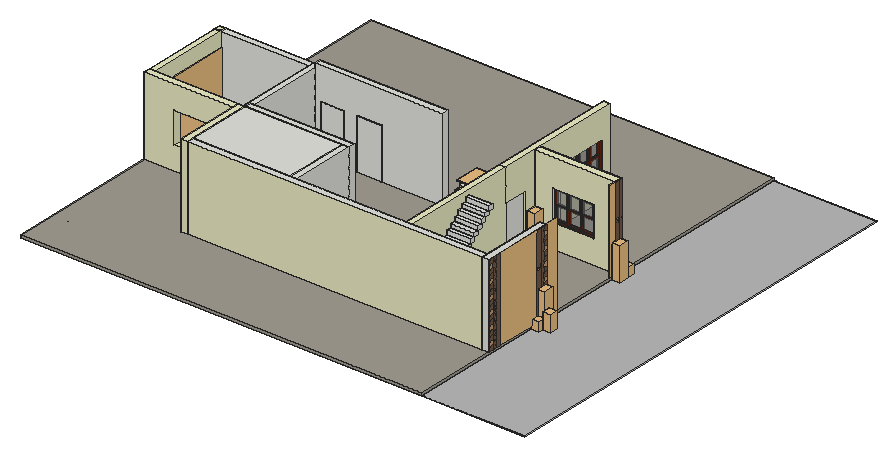
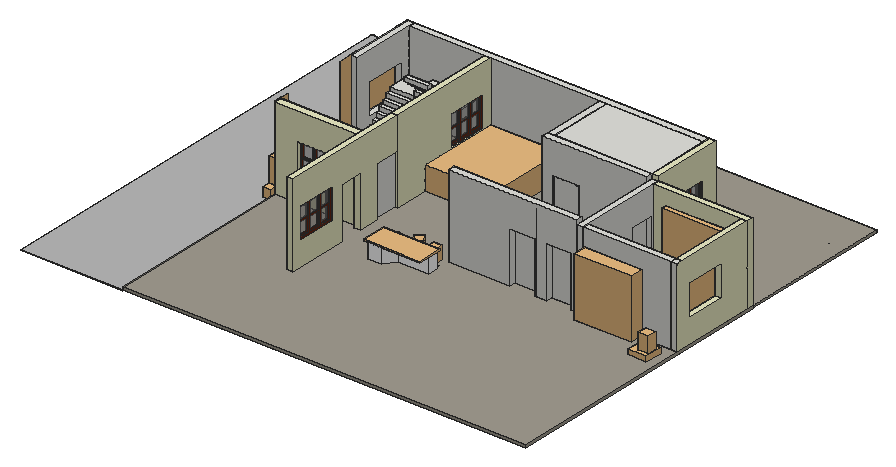
# SketchUp Ruby script. Lengths in inches.
U = 1.inch
M = Sketchup.active_model
def pt(a) = Geom::Point3d.new(a.map { |v| v * U })
def face(e, loops, mat)
  f = e.add_face(loops[0].map { |a| pt(a) })
  loops[1..].each { |l| e.add_face(l.map { |a| pt(a) }).erase! }
  f.material = f.back_material = mat if mat
  f
end
# faces: each face lists its corners as indices into pts; further lists are holes
def faces(e, pts, list, mat = nil) = list.each { |f| face(e, (f[0].is_a?(Array) ? f : [f]).map { |l| l.map { |i| pts[i] } }, mat) }
# xy, xz, yz: faces in a plane at the given z, y or x. An outline is a flat list of corners, or four numbers for a rectangle; further outlines are holes
def ring(l) = l.size == 4 ? [[l[0], l[1]], [l[2], l[1]], [l[2], l[3]], [l[0], l[3]]] : l.each_slice(2).to_a
def flat(e, list, mat, &to3) = list.each { |f| face(e, (f[0].is_a?(Array) ? f : [f]).map { |l| ring(l).map { |u, v| to3.(u, v) } }, mat) }
def xy(e, z, list, mat = nil) = flat(e, list, mat) { |x, y| [x, y, z] }
def xz(e, y, list, mat = nil) = flat(e, list, mat) { |x, z| [x, y, z] }
def yz(e, x, list, mat = nil) = flat(e, list, mat) { |y, z| [x, y, z] }
def lines(e, pts, list) = list.each { |a, b| e.add_line(pt(pts[a]), pt(pts[b])) }
# prism: a flat outline (further loops are holes) pulled along v
def prism(e, loops, v, mat = nil)
  f = face(e, loops, mat); d = Geom::Vector3d.new(v.map { |x| x * U })
  f.pushpull(f.normal.samedirection?(d) ? d.length : -d.length)
end
def box(e, o, s, mat = nil) = prism(e, [[o, [o[0] + s[0], o[1], o[2]], [o[0] + s[0], o[1] + s[1], o[2]], [o[0], o[1] + s[1], o[2]]]], [0, 0, s[2]], mat)
def at(x, y, z, deg = 0) = Geom::Transformation.translation(pt([x, y, z])) * Geom::Transformation.rotation(ORIGIN, Z_AXIS, deg.degrees)
def axes(o, x, y, z) = Geom::Transformation.new([*x, 0, *y, 0, *z, 0, *pt(o).to_a, 1])
def part(name) = M.definitions.add(name)
# library, detail: a bought-in or finely detailed component or shape, given as its bounding box
def library(name, o, s) = part(name).tap { |d| box(d.entities, o, s) }
def detail(e, o, s) = box(e.add_group.entities, o, s)
def put(e, d, t, mat = nil) = e.add_instance(d, t).tap { |i| i.material = mat if mat }
def group(e, t, mat = nil) = e.add_group.tap { |g| g.transformation = t; g.material = mat if mat }.entities
root = M.entities
M.materials.add("02 - Default1").color = [198, 154, 113]
M.materials.add("1").color = [234, 234, 196]
M.materials.add("3").color = [118, 89, 74]
M.materials.add("6").color = [162, 157, 145]
M.materials.add("Material1 glass").color = [170, 237, 177]
M.materials["Material1 glass"].alpha = 0.04
M.materials.add("Material1 metal").color = [192, 192, 192]
M.materials.add("[0080_DarkCyan]").color = [185, 185, 185]
M.materials.add("[Carpet_Plush_Charcoal]1").color = [87, 87, 87]
M.materials.add("[Color_004]1").color = [142, 142, 142]
M.materials.add("[Color_005]").color = [114, 114, 114]
M.materials.add("[Color_B17]").color = [102, 40, 20]
M.materials.add("[Tile_Ceramic_Natural]").color = [73, 73, 73]
M.materials.add("[Tile_Ceramic_Natural]1").color = [234, 234, 234]
M.materials.add("[Translucent_Glass_Gray]").color = [128, 128, 128]
M.materials["[Translucent_Glass_Gray]"].alpha = 0.5
M.materials.add("[Wood_ Floor]").color = [155, 105, 61]
M.materials.add("[Wood_Lumber_ButtJoined]").color = [69, 62, 43]
M.materials.add("putih ceramic").color = [255, 255, 255]
c1 = part("Group\#331")
xy(c1.entities,0,[[0,0,0.82,6.2]],"1")
xy(c1.entities,114.11,[[0,0,0.82,6.2]],"1")
xz(c1.entities,0,[[0,0,0.82,114.11]],"1")
xz(c1.entities,6.2,[[0,0,0.82,114.11]],"1")
yz(c1.entities,0,[[0,0,6.2,114.11]],"1")
yz(c1.entities,0.82,[[0,0,6.2,114.11]],"3")
c2 = part("Group\#330")
put(c2.entities,c1,axes([-0.82,0,0],[1,0,0],[0,1.45243,0],[0,0,1]),"1")
c3 = part("Group\#329")
box(c3.entities,[0,0,0],[0.82,6.2,114.11],"02 - Default1")
c4 = part("Group\#328")
put(c4.entities,c3,axes([-0.82,0,0],[1,0,0],[0,1.45243,0],[0,0,1]))
c5 = part("Group\#286")
put(c5.entities,c2,axes([0.82,0,0],[1,0,0],[0,0.6885,0],[0,0,1]),"02 - Default1")
put(c5.entities,c2,axes([0.82,6.2,89.22],[1,0,0],[0,0,0.67033],[0,-0.05434,0]),"02 - Default1")
put(c5.entities,c2,axes([0.82,6.2,12.68],[1,0,0],[0,0,0.67033],[0,-0.05434,0]),"02 - Default1")
put(c5.entities,c4,axes([0.82,6.2,63.7],[1,0,0],[0,0,0.67033],[0,-0.05434,0]),"02 - Default1")
put(c5.entities,c4,axes([0.82,6.2,25.75],[1,0,0],[0,0,0.67033],[0,-0.05434,0]),"02 - Default1")
put(c5.entities,c4,axes([0.82,6.2,82.99],[1,0,0],[0,0,0.67033],[0,-0.05434,0]),"02 - Default1")
put(c5.entities,c2,axes([0.82,6.2,50.83],[1,0,0],[0,0,0.67033],[0,-0.05434,0]),"02 - Default1")
put(c5.entities,c2,axes([0.82,6.2,76.54],[1,0,0],[0,0,0.67033],[0,-0.05434,0]),"02 - Default1")
put(c5.entities,c2,axes([0.82,6.2,31.98],[1,0,0],[0,0,0.67033],[0,-0.05434,0]),"02 - Default1")
put(c5.entities,c4,axes([0.82,6.2,44.6],[1,0,0],[0,0,0.67033],[0,-0.05434,0]),"02 - Default1")
g1 = group(c5.entities,at(0.82,6.2,95.39),"02 - Default1")
put(g1,c1,axes([-0.82,0,0],[1,0,0],[0,0,0.97361],[0,-0.05434,0]),"1")
put(c5.entities,c4,axes([0.82,6.2,101.84],[1,0,0],[0,0,0.67033],[0,-0.05434,0]),"02 - Default1")
put(c5.entities,c2,axes([0.82,6.2,0],[1,0,0],[0,0,0.67033],[0,-0.05434,0]),"02 - Default1")
put(c5.entities,c2,axes([0.82,6.2,19.3],[1,0,0],[0,0,0.67033],[0,-0.05434,0]),"02 - Default1")
put(c5.entities,c2,axes([0.82,6.2,69.93],[1,0,0],[0,0,0.67033],[0,-0.05434,0]),"02 - Default1")
put(c5.entities,c4,axes([0.82,6.2,6.45],[1,0,0],[0,0,0.67033],[0,-0.05434,0]),"02 - Default1")
put(c5.entities,c2,axes([0.82,6.2,38.15],[1,0,0],[0,0,0.67033],[0,-0.05434,0]),"02 - Default1")
put(c5.entities,c2,axes([0.82,6.2,57.25],[1,0,0],[0,0,0.67033],[0,-0.05434,0]),"02 - Default1")
put(c5.entities,c2,axes([0.82,6.2,108.07],[1,0,0],[0,0,0.67033],[0,-0.05434,0]),"02 - Default1")
c6 = library("Group\#185",[0,0,0],[15.75,57.83,12.57])
c7 = library("Group\#183",[0,0,0],[15.75,57.83,12.57])
c8 = library("Toilet",[49.48,5.86,0],[19.92,29.67,40.01])
c9 = library("Group\#134",[0,0,0],[3.17,3.17,3.01])
c10 = part("Framed panel")
g2 = group(c10.entities,at(0,0,0))
prism(g2,[[[0,22.64,0],[21.26,22.64,0],[21.26,0,0],[0,0,0]],[[1.57,1.57,0],[19.69,1.57,0],[19.69,21.0625,0],[1.57,21.0625,0]]],[0,0,1.57],"[Color_B17]")
g3 = group(c10.entities,at(1.57,1.57,1.02))
xy(g3,0,[[0,0,18.11,19.49]],"[Translucent_Glass_Gray]")
c11 = part("Group\#25")
put(c11.entities,c10,at(0,21.0625,1.57))
put(c11.entities,c10,at(0,0,0))
c12 = part("Group\#47")
g4 = group(c12.entities,at(0,0,0))
prism(g4,[[[70.87,0,0],[0,0,0],[0,47.24,0],[70.87,47.24,0]],[[47.83,1.77,0],[69.09,1.77,0],[69.09,45.47,0],[47.83,45.47,0]],[[46.0625,45.47,0],[24.8,45.47,0],[24.8,1.77,0],[46.0625,1.77,0]],[[1.77,1.77,0],[23.03,1.77,0],[23.03,45.47,0],[1.77,45.47,0]]],[0,0,4.33],"[Color_B17]")
put(c12.entities,c11,at(1.77,1.77,0.59))
put(c12.entities,c11,at(24.8,1.77,0.59))
put(c12.entities,c11,at(47.83,1.77,0.59))
c13 = library("Group\#332",[0,0,0],[0.82,72.71,126.79])
c14 = part("Group\#195")
box(c14.entities,[0,-29,0],[36,36,6])
c15 = part("Group\#196")
box(c15.entities,[0,0,0],[36,7,6])
c16 = part("Group\#197")
box(c16.entities,[0,0,0],[36,7,6])
c17 = part("Group\#165")
xy(c17.entities,0,[[3.14,0.77,2.7,0.83,2.28,1,1.93,1.27,1.65,1.63,1.48,2.04,4.8,2.93,4.86,2.49,4.8,2.04,4.63,1.63,4.36,1.27,4,1,3.59,0.83],[24.03,0.77,23.59,0.83,23.17,1,22.81,1.27,22.54,1.63,25.25,3.7,25.52,3.35,25.69,2.93,25.75,2.49,25.69,2.04,25.52,1.63,25.25,1.27,24.89,1,24.48,0.83],[22.54,1.63,22.37,2.04,22.3125,2.49,22.37,2.93,22.54,3.35,22.81,3.7,23.17,3.98,23.59,4.15,24.03,4.21,24.48,4.15,24.89,3.98,25.25,3.7],[1.48,2.04,1.42,2.49,1.48,2.93,1.65,3.35,1.93,3.7,2.28,3.98,2.7,4.15,3.14,4.21,3.59,4.15,4,3.98,4.36,3.7,4.63,3.35,4.8,2.93]],"[Color_005]")
xy(c17.entities,2.2,[[3.14,0.77,3.59,0.83,4,1,4.36,1.27,4.63,1.63,4.8,2.04,4.86,2.49,4.8,2.93,4.63,3.35,4.36,3.7,4,3.98,3.59,4.15,3.14,4.21,2.7,4.15,2.28,3.98,1.93,3.7,1.65,3.35,1.48,2.93,1.42,2.49,1.48,2.04,1.65,1.63,1.93,1.27,2.28,1,2.7,0.83],[24.03,0.77,24.48,0.83,24.89,1,25.25,1.27,25.52,1.63,25.69,2.04,25.75,2.49,25.69,2.93,25.52,3.35,25.25,3.7,24.89,3.98,24.48,4.15,24.03,4.21,23.59,4.15,23.17,3.98,22.81,3.7,22.54,3.35,22.37,2.93,22.3125,2.49,22.37,2.04,22.54,1.63,22.81,1.27,23.17,1,23.59,0.83]])
p = [[2.28,1,0],[2.7,0.83,0],[2.7,0.83,2.2],[2.28,1,2.2],[3.14,0.77,0],[3.14,0.77,2.2],
  [3.59,0.83,0],[3.59,0.83,2.2],[4,1,0],[4,1,2.2],[23.17,1,0],[23.59,0.83,0],
  [23.59,0.83,2.2],[23.17,1,2.2],[24.03,0.77,0],[24.03,0.77,2.2],[24.48,0.83,0],[24.48,0.83,2.2],
  [24.89,1,0],[24.89,1,2.2],[1.93,1.27,0],[1.93,1.27,2.2],[4.36,1.27,0],[4.36,1.27,2.2],
  [22.81,1.27,0],[22.81,1.27,2.2],[25.25,1.27,0],[25.25,1.27,2.2],[1.65,1.63,0],[1.65,1.63,2.2],
  [4.63,1.63,0],[4.63,1.63,2.2],[22.54,1.63,0],[22.54,1.63,2.2],[25.52,1.63,0],[25.52,1.63,2.2],
  [1.48,2.04,0],[1.48,2.04,2.2],[4.8,2.04,0],[4.8,2.04,2.2],[22.37,2.04,0],[22.37,2.04,2.2],
  [25.69,2.04,0],[25.69,2.04,2.2],[1.42,2.49,0],[1.42,2.49,2.2],[4.86,2.49,0],[4.86,2.49,2.2],
  [22.3125,2.49,0],[22.3125,2.49,2.2],[25.75,2.49,0],[25.75,2.49,2.2],[1.48,2.93,0],[1.48,2.93,2.2],
  [4.8,2.93,0],[4.8,2.93,2.2],[22.37,2.93,0],[22.37,2.93,2.2],[25.69,2.93,0],[25.69,2.93,2.2],
  [1.65,3.35,0],[1.65,3.35,2.2],[4.63,3.35,0],[4.63,3.35,2.2],[22.54,3.35,0],[22.54,3.35,2.2],
  [25.52,3.35,0],[25.52,3.35,2.2],[1.93,3.7,0],[1.93,3.7,2.2],[4.36,3.7,0],[4.36,3.7,2.2],
  [22.81,3.7,0],[22.81,3.7,2.2],[25.25,3.7,0],[25.25,3.7,2.2],[2.28,3.98,0],[2.28,3.98,2.2],
  [4,3.98,0],[4,3.98,2.2],[23.17,3.98,0],[23.17,3.98,2.2],[24.89,3.98,0],[24.89,3.98,2.2],
  [2.7,4.15,0],[2.7,4.15,2.2],[3.59,4.15,0],[3.59,4.15,2.2],[23.59,4.15,0],[23.59,4.15,2.2],
  [24.48,4.15,0],[24.48,4.15,2.2],[3.14,4.21,0],[3.14,4.21,2.2],[24.03,4.21,0],[24.03,4.21,2.2]]
faces(c17.entities,p,[[0,1,2,3],[1,4,5,2],[4,6,7,5],[6,8,9,7],[10,11,12,13],[11,14,15,12],[14,16,17,15],[16,18,19,17],
  [20,0,3,21],[8,22,23,9],[24,10,13,25],[18,26,27,19],[28,20,21,29],[22,30,31,23],[32,24,25,33],[26,34,35,27],
  [36,28,29,37],[30,38,39,31],[40,32,33,41],[34,42,43,35],[44,36,37,45],[38,46,47,39],[48,40,41,49],[42,50,51,43],
  [52,44,45,53],[46,54,55,47],[56,48,49,57],[50,58,59,51],[60,52,53,61],[54,62,63,55],[64,56,57,65],[58,66,67,59],
  [68,60,61,69],[62,70,71,63],[72,64,65,73],[66,74,75,67],[76,68,69,77],[70,78,79,71],[80,72,73,81],[74,82,83,75],
  [84,76,77,85],[78,86,87,79],[88,80,81,89],[82,90,91,83],[92,84,85,93],[86,92,93,87],[94,88,89,95],[90,94,95,91]],"[Color_005]")
g5 = group(c17.entities,at(0,0,1.83),"[Color_005]")
box(g5,[0,0,0],[27.7,4.93,1.59])
c18 = library("Group\#192",[0,0,0],[140.56,162.1,33.05])
c19 = library("Agrupar\#4",[0,0.16,0],[12.11,12.1,27.76])
c20 = library("Agrupar\#6",[0,0,0],[12.11,12.11,39.78])
c21 = library("Agrupar\#5",[-0.57,-0.61,0],[12.2,15.09,63.23])
c22 = library("Group\#226",[0,0,-2.65],[191.01,383.01,2.65])
c23 = part("DOOR12")
g6 = group(c23.entities,at(114.73,28.14,-0.51))
g7 = group(g6,at(0,0,0))
box(g7,[0,0,0],[36,0.5,77.7])
c24 = library("Window curtains 2",[0,-81.89,0],[92,82.37,8.12])
c25 = library("Dressing_table",[0,-6.3125,-0.01],[54.59,27.125,100.87])
c26 = part("Group\#193")
prism(c26.entities,[[[0,134,120],[0,134,0],[0,41,0],[0,41,78],[0,2,78],[0,2,0],[0,-10,0],[0,-10,120]]],[10,0,0])
c27 = library("mesh-256",[-120.04,-169.59,0.14],[253.19,307.8,1.7])
c28 = part("Group7")
put(c28.entities,c27,at(0,0,0))
c29 = library("Group10",[-94.75,-3.97,0],[199.87,106.11,39.4375])
c30 = library("mesh-258",[-96.03,-121.28,21.97],[201.42,163.89,40.48])
c31 = library("Group14",[-46.92,-34.29,0],[94.87,68.58,31.875])
c32 = library("Group16",[-47.82,-34.55,0],[96.75,69.58,33.34])
c33 = library("Group18",[-33.62,-26.58,0],[67.24,53.16,20.44])
c34 = library("Group20",[-0.01,-0.01,0.02],[107.76,124.16,6.31])
c35 = library("mesh-263",[-97.08,-118.58,12.75],[201.41,233.93,94.93])
c36 = library("mesh-264",[-106.11,-80.86,12.52],[217.88,74.95,54.44])
c37 = part("Group9")
put(c37.entities,c29,axes([-2.83,3.64,23.125],[0.96274,0,0],[0,0.96274,0],[0,0,0.96274]))
g8 = group(c37.entities,at(-2.83,3.64,23.41))
put(g8,c30,axes([0,0,-21.09],[0.96274,0,0],[0,0.96274,0],[0,0,0.96274]))
put(c37.entities,c31,at(49.15,58.47,50.125))
put(c37.entities,c32,at(-47.3,60.89,49.06))
put(c37.entities,c33,at(-22.74,14.21,61.08))
put(c37.entities,c34,axes([-96.54,-113.26,0],[1.80992,0,0],[0,1.80992,0],[0,0,1.80992]))
g9 = group(c37.entities,at(-2.83,1.61,11.33))
put(g9,c35,at(0,0,-12.75))
g10 = group(c37.entities,at(-2.83,20.36,11.1))
put(g10,c36,at(0,0,-12.52))
c38 = library("Group26",[-8.72,-28.73,0.18],[47.65,50.07,77.26])
c39 = library("Group",[-44.49,-44.49,0],[88.98,89.04,25.37])
c40 = library("Group\#231",[0,0,-2.65],[191.01,383.01,2.65])
c41 = part("Group\#94")
xz(c41.entities,0,[[0,0,144,120]])
g11 = group(c41.entities,at(0,0,0))
yz(g11,0,[[0,0,10,120]])
p = [[0,0,120],[134,0,120],[134,0,0],[0,0,0]]
lines(g11,p,[[0,1],[2,3]])
g12 = group(g11,at(0,0,0))
xy(g12,0,[[0,0,144,10]])
xy(g12,120,[[0,0,144,10]])
xz(g12,10,[[0,0,144,120]])
yz(g12,144,[[0,0,10,120]])
c42 = library("HMI+SHE+SAID+BARSTOOL",[-9.1,-9.7,0],[19.23,19.64,34.25])
c43 = library("wardrobe",[25.55,74.38,0],[101.97,24.01,104.72])
c44 = part("Component\#31")
prism(c44.entities,[[[0,0.17,1.01],[0,0.3,1.1],[0,0.4375,1.16],[0,0.59,1.18],[0,0.74,1.16],[0,0.89,1.1],[0,1.01,1.01],[0,1.1,0.89],[0,1.16,0.74],[0,1.18,0.59],[0,1.16,0.4375],[0,1.1,0.3],[0,1.01,0.17],[0,0.89,0.08],[0,0.74,0.02],[0,0.59,0],[0,0.4375,0.02],[0,0.3,0.08],[0,0.17,0.17],[0,0.08,0.3],[0,0.02,0.4375],[0,0,0.59],[0,0.02,0.74],[0,0.08,0.89]]],[0.2,0,0],"Material1 metal")
c45 = part("Component\#21")
box(c45.entities,[0,0,0],[0.59,79.03,0.79],"putih ceramic")
c46 = part("Component\#33")
prism(c46.entities,[[[0.91,0.01,0.74],[0.87,0.05,0.89],[0.79,0.11,1.01],[0.7,0.18,1.1],[0.58,0.27,1.16],[0.46,0.36,1.18],[0.34,0.46,1.16],[0.23,0.55,1.1],[0.14,0.62,1.01],[0.0625,0.68,0.89],[0.02,0.72,0.74],[0,0.73,0.59],[0.02,0.72,0.4375],[0.0625,0.68,0.3],[0.14,0.62,0.17],[0.23,0.55,0.08],[0.34,0.46,0.02],[0.46,0.36,0],[0.58,0.27,0.02],[0.7,0.18,0.08],[0.79,0.11,0.17],[0.87,0.05,0.3],[0.91,0.01,0.4375],[0.93,0,0.59]]],[0.12,0.15,0],"Material1 metal")
c47 = part("Component\#24")
xy(c47.entities,0,[[0,0,0.39,78.5]],"Material1 glass")
xy(c47.entities,27.95,[[0,0,0.39,78.5]],"Material1 glass")
xz(c47.entities,0,[[0,0,0.39,27.95]],"Material1 glass")
xz(c47.entities,78.5,[[0,0,0.39,27.95]],"Material1 glass")
yz(c47.entities,0.39,[[0,0,78.5,27.95]],"Material1 glass")
c48 = library("Component\#2",[0,0,0],[54.72,125.67,2.36])
c49 = part("Component\#28")
xy(c49.entities,0,[[46.66,-0.1,0,36.57,0.24,36.88,46.91,0.21]],"Material1 glass")
xy(c49.entities,27.95,[[46.66,-0.1,46.91,0.21,0.24,36.88,0,36.57]],"Material1 glass")
p = [[46.91,0.21,0],[46.91,0.21,27.95],[46.66,-0.1,27.95],[46.66,-0.1,0],[0.24,36.88,27.95],[0.24,36.88,0],
  [0,36.57,0],[0,36.57,27.95]]
faces(c49.entities,p,[[0,1,2,3],[4,1,0,5],[4,5,6,7]],"Material1 glass")
c50 = part("Component\#27")
prism(c50.entities,[[[46.85,0,0],[23.23,0,0],[23.23,67.26,0],[0,85.51,0],[0,115.55,0],[46.85,78.74,0]]],[0,0,33.07],"putih ceramic")
xy(root,-4.79,[[1942.8125,0,2100.39,671.39]])
xy(root,-4,[[1942.8125,0,2100.39,671.39]],"[0080_DarkCyan]")
xy(root,0,[[1481.72,126.94,1932.8125,137.4],[1932.8125,126.94,1942.8125,236.85],[1630.57,137.4,1641.41,236.85]])
xy(root,0,[[1481.72,137.4,1619.11,148.45],[1619.11,137.4,1630.57,236.85]],"[Tile_Ceramic_Natural]")
xy(root,0,[[1481.72,148.45,1619.11,236.85]],"[Tile_Ceramic_Natural]1")
xy(root,36,[[1932.8125,151.95,1942.8125,213.95]])
xy(root,84,[[1932.8125,151.95,1942.8125,213.95]])
xy(root,126.79,[[1481.72,126.94,1932.8125,137.4],[1932.8125,126.94,1942.8125,236.85],[1481.72,137.4,1630.57,236.85],[1630.57,137.4,1641.41,236.85]])
xz(root,0,[[1942.8125,-4.79,2100.39,-4]])
xz(root,126.94,[[1932.8125,0,1942.8125,126.79]])
xz(root,126.94,[[1481.72,0,1932.8125,126.79]],"1")
xz(root,137.4,[[1630.57,0,1641.41,126.79],[1641.41,0,1932.8125,126.79]])
xz(root,137.4,[[1575.05,0,1594.72,126.79]],"[Tile_Ceramic_Natural]")
xz(root,137.4,[[1481.72,0,1575.05,126.79],[1594.72,0,1630.57,126.79]],"[Tile_Ceramic_Natural]1")
xz(root,151.95,[[1932.8125,36,1942.8125,84]])
xz(root,213.95,[[1932.8125,36,1942.8125,84]])
xz(root,236.85,[[1630.57,0,1641.41,126.79],[1932.8125,0,1942.8125,126.79],[1481.72,120,1630.57,126.79]])
xz(root,671.39,[[1942.8125,-4.79,2100.39,-4]])
yz(root,1481.72,[[126.94,0,137.4,126.79],[137.4,120,236.85,126.79]])
yz(root,1630.57,[[163.97,6.73,174.04,35.43],[174.04,6.73,199.83,35.43],[199.83,6.73,211.45,35.43]])
yz(root,1630.57,[[174.04,0,199.83,6.73],[174.04,35.43,199.83,126.79]],"[Tile_Ceramic_Natural]")
yz(root,1630.57,[[137.4,0,137.4,126.79,174.04,126.79,174.04,35.43,163.97,35.43,163.97,6.73,174.04,6.73,174.04,0],[199.83,0,199.83,6.73,211.45,6.73,211.45,35.43,199.83,35.43,199.83,126.79,236.85,126.79,236.85,0]],"[Tile_Ceramic_Natural]1")
yz(root,1641.41,[[137.4,0,236.85,126.79]])
yz(root,1932.8125,[[126.94,0,137.4,126.79],[[137.4,0,236.85,126.79],[151.95,36,213.95,84]]])
yz(root,1942.8125,[[0,-4.79,671.39,-4],[[126.94,0,236.85,126.79],[151.95,36,213.95,84]]])
yz(root,2100.39,[[0,-4.79,671.39,-4]])
p = [[1731.85,399.4375,3.26],[1731.85,399.4375,2.72],[1732.17,399.19,2.72],[1732.17,399.19,3.26],[1543.51,380.85,0],[1543.51,380.85,120],
  [1471.72,246.85,0],[1471.72,246.85,120],[1327.72,246.85,0],[1350.8125,62.53,0],[1350.2,62.53,0],[1731.97,399.59,3.26]]
faces(root,p,[[0,1,2,3]],"putih ceramic")
lines(root,p,[[4,5],[6,7],[8,6],[9,10],[11,0]])
put(root,c5,axes([1942.8125,127.88,0],[1,0,0],[0,1,0],[0,0,1.11]))
put(root,c5,axes([1942.8125,134.08,0],[1,0,0],[0,1,0],[0,0,1.11]))
g13 = group(root,at(1540.7,137.42,0))
xy(g13,0,[[-15.13,0,0,5.36]])
xy(g13,10.45,[[-15.13,0,0,5.36]])
xz(g13,0,[[-15.13,0,0,10.45]])
xz(g13,5.36,[[-15.13,0,0,3.85],[-15.13,3.85,0,10.45]])
yz(g13,-15.13,[[0,0,5.36,3.85],[0,3.85,5.36,10.45]])
yz(g13,0,[[0,0,5.36,3.85],[0,3.85,5.36,10.45]])
put(root,c5,axes([1942.8125,140.28,0],[1,0,0],[0,1,0],[0,0,1.11]))
put(root,c6,axes([1583.96,137.4,6.73],[-1,0,0],[0,0,1],[0,1,0]),"[Wood_Lumber_ButtJoined]")
put(root,c7,axes([1602.34,137.52,6.73],[-1,0,0],[0,0,1],[0,1,0]))
put(root,c8,at(1454.32,131.54,0))
g14 = group(root,at(1586.49,158,0),"[Color_004]1")
xy(g14,17.37,[[-3.04,-3.33,-2.96,-3.33,-2.875,-3.31,-2.8,-3.26,-2.74,-3.2,-2.7,-3.125,-2.68,-3.04,-2.68,-2.96,-2.71,-2.875,-2.75,-2.8,-2.8125,-2.74,-2.89,-2.7,-2.97,-2.68,-3.06,-2.68,-3.14,-2.71,-3.21,-2.75,-3.27,-2.8125,-3.3125,-2.89,-3.33,-2.97,-3.33,-3.06,-3.31,-3.14,-3.26,-3.21,-3.2,-3.27,-3.125,-3.3125]])
g15 = group(g14,at(-2.68,-2.68,1.0625))
xz(g15,-0.65,[[-0.36,0,-0.28,16.31]])
xz(g15,0,[[-0.375,0,-0.29,16.31]])
yz(g15,-0.65,[[-0.375,0,-0.29,16.31]])
yz(g15,0,[[-0.36,0,-0.28,16.31]])
p = [[-0.44,-0.63,0],[-0.36,-0.65,0],[-0.36,-0.65,16.31],[-0.44,-0.63,16.31],[-0.58,-0.53,0],[-0.52,-0.59,0],
  [-0.52,-0.59,16.31],[-0.58,-0.53,16.31],[-0.28,-0.65,0],[-0.19,-0.625,0],[-0.19,-0.625,16.31],[-0.28,-0.65,16.31],
  [-0.12,-0.58,0],[-0.12,-0.58,16.31],[-0.0625,-0.52,0],[-0.0625,-0.52,16.31],[-0.625,-0.46,0],[-0.625,-0.46,16.31],
  [-0.65,-0.375,0],[-0.65,-0.375,16.31],[-0.02,-0.44,0],[-0.02,-0.44,16.31],[0,-0.36,0],[0,-0.36,16.31],
  [-0.63,-0.21,0],[-0.65,-0.29,0],[-0.65,-0.29,16.31],[-0.63,-0.21,16.31],[0,-0.28,0],[-0.03,-0.19,0],
  [-0.03,-0.19,16.31],[0,-0.28,16.31],[-0.59,-0.13,0],[-0.59,-0.13,16.31],[-0.07,-0.12,0],[-0.07,-0.12,16.31],
  [-0.53,-0.07,0],[-0.53,-0.07,16.31],[-0.46,-0.03,0],[-0.46,-0.03,16.31],[-0.13,-0.0625,0],[-0.21,-0.02,0],
  [-0.21,-0.02,16.31],[-0.13,-0.0625,16.31],[-0.375,0,0],[-0.375,0,16.31],[-0.29,0,0],[-0.29,0,16.31]]
faces(g15,p,[[0,1,2,3],[4,5,6,7],[5,0,3,6],[8,9,10,11],[9,12,13,10],[12,14,15,13],[16,4,7,17],[18,16,17,19],
  [14,20,21,15],[20,22,23,21],[24,25,26,27],[28,29,30,31],[32,24,27,33],[29,34,35,30],[36,32,33,37],[38,36,37,39],
  [40,41,42,43],[34,40,43,35],[44,38,39,45],[41,46,47,42]])
g16 = group(g14,at(0,0,0))
detail(g16,[-6.01,-6.01,0],[6.01,6.01,1.0625])
put(root,c9,axes([1531.68,153.5,4.7],[-1,0,0],[0,1,0],[0,0,-1.20757]))
put(root,c9,axes([1531.68,153.5,8.35],[-1,0,0],[0,1,0],[0,0,-1.20757]))
put(root,c9,axes([1531.68,153.5,12.01],[-1,0,0],[0,1,0],[0,0,-1.20757]))
put(root,c9,axes([1531.68,153.5,15.71],[-1,0,0],[0,1,0],[0,0,-1.20757]))
g17 = group(root,at(1471.72,124.98,0),"1")
g18 = group(g17,at(0,111.87,0,-90))
xy(g18,0,[[0,0,109.91,10]])
xy(g18,36,[[22.9,0,84.9,10]])
xy(g18,84,[[22.9,0,84.9,10]])
xy(g18,126.79,[[0,0,109.91,10]])
xz(g18,0,[[[0,0,109.91,126.79],[22.9,36,84.9,84]]])
xz(g18,10,[[[0,0,109.91,126.79],[22.9,36,84.9,84]]])
yz(g18,0,[[0,0,10,126.79]])
yz(g18,22.9,[[0,36,10,84]])
yz(g18,84.9,[[0,36,10,84]])
yz(g18,109.91,[[0,0,10,126.79]])
put(g17,c12,axes([6.625,88.97,36],[0,-0.87489,0],[0,0,1.016],[-1,0,0]))
put(root,c13,at(1942.8125,146.25,0))
g19 = group(root,at(1607.87,208.66,0,-180))
xy(g19,0,[[19.32,0,13.75,1.39,8.74,4.18,4.62,8.17,1.67,13.09,0.09,18.6,0,24.34,1.39,29.9,4.18,34.92,8.17,39.04,13.09,41.99,18.6,43.5625,24.34,43.66,29.9,42.26,34.92,39.48,39.04,35.49,41.99,30.57,43.5625,25.05,43.66,19.32,42.26,13.75,39.48,8.74,35.49,4.62,30.57,1.67,25.05,0.09]])
xy(g19,0.23,[[19.32,0,25.05,0.09,30.57,1.67,35.49,4.62,39.48,8.74,42.26,13.75,43.66,19.32,43.5625,25.05,41.99,30.57,39.04,35.49,34.92,39.48,29.9,42.26,24.34,43.66,18.6,43.5625,13.09,41.99,8.17,39.04,4.18,34.92,1.39,29.9,0,24.34,0.09,18.6,1.67,13.09,4.62,8.17,8.74,4.18,13.75,1.39]],"[Carpet_Plush_Charcoal]1")
p = [[13.75,1.39,0],[19.32,0,0],[19.32,0,0.23],[13.75,1.39,0.23],[25.05,0.09,0],[25.05,0.09,0.23],
  [30.57,1.67,0],[30.57,1.67,0.23],[8.74,4.18,0],[8.74,4.18,0.23],[35.49,4.62,0],[35.49,4.62,0.23],
  [4.62,8.17,0],[4.62,8.17,0.23],[39.48,8.74,0],[39.48,8.74,0.23],[1.67,13.09,0],[1.67,13.09,0.23],
  [42.26,13.75,0],[42.26,13.75,0.23],[0.09,18.6,0],[0.09,18.6,0.23],[43.66,19.32,0],[43.66,19.32,0.23],
  [0,24.34,0],[0,24.34,0.23],[43.5625,25.05,0],[43.5625,25.05,0.23],[1.39,29.9,0],[1.39,29.9,0.23],
  [41.99,30.57,0],[41.99,30.57,0.23],[4.18,34.92,0],[4.18,34.92,0.23],[39.04,35.49,0],[39.04,35.49,0.23],
  [8.17,39.04,0],[8.17,39.04,0.23],[34.92,39.48,0],[34.92,39.48,0.23],[13.09,41.99,0],[13.09,41.99,0.23],
  [29.9,42.26,0],[29.9,42.26,0.23],[18.6,43.5625,0],[18.6,43.5625,0.23],[24.34,43.66,0],[24.34,43.66,0.23]]
faces(g19,p,[[0,1,2,3],[1,4,5,2],[4,6,7,5],[8,0,3,9],[6,10,11,7],[12,8,9,13],[10,14,15,11],[16,12,13,17],
  [14,18,19,15],[20,16,17,21],[18,22,23,19],[24,20,21,25],[22,26,27,23],[28,24,25,29],[26,30,31,27],[32,28,29,33],
  [30,34,35,31],[36,32,33,37],[34,38,39,35],[40,36,37,41],[38,42,43,39],[44,40,41,45],[42,46,47,43],[46,44,45,47]],"[Carpet_Plush_Charcoal]1")
g20 = group(root,at(1824.8125,137.85,0))
put(g20,c14,at(72,29,54))
put(g20,c15,at(72,36,48))
put(g20,c15,at(72,43,42))
put(g20,c15,at(72,50,36))
put(g20,c16,at(0,36,72))
put(g20,c14,at(36,29,60))
put(g20,c14,at(0,29,66))
put(g20,c16,at(0,43,78))
put(g20,c16,at(0,92,120))
put(g20,c16,at(0,57,90))
put(g20,c16,at(0,50,84))
put(g20,c16,at(0,64,96))
put(g20,c16,at(0,71,102))
put(g20,c16,at(0,78,108))
put(g20,c16,at(0,85,114))
put(g20,c15,at(72,92,0))
put(g20,c15,at(72,78,12))
put(g20,c15,at(72,85,6))
put(g20,c15,at(72,64,24))
put(g20,c15,at(72,71,18))
put(g20,c15,at(72,57,30))
put(root,c17,axes([1618.76,192.77,15.01],[0,-0.3762,0],[0,0,0.25582],[-0.3762,0,0]))
g21 = group(root,at(1630.57,211.45,6.73,-180),"[Wood_ Floor]")
xy(g21,0,[[0,0,11.42,0,11.42,0.2,11.46,0.2,11.46,0,11.8125,0,11.8125,47.48,11.46,47.48,11.46,47.28,11.42,47.28,11.42,47.48,0,47.48]],"[Wood_Lumber_ButtJoined]")
xy(g21,11.24,[[11.46,0,11.46,0.2,11.42,0.2,11.42,47.28,11.46,47.28,11.46,47.48,11.8125,47.48,11.8125,0]],"[Wood_Lumber_ButtJoined]")
xy(g21,11.36,[[11.46,0,11.8125,0,11.8125,47.48,11.46,47.48,11.46,47.28,11.42,47.28,11.42,0.2,11.46,0.2]],"[Wood_Lumber_ButtJoined]")
xy(g21,20.26,[[11.46,0,11.46,0.2,11.42,0.2,11.42,47.28,11.46,47.28,11.46,47.48,11.8125,47.48,11.8125,0]],"[Wood_Lumber_ButtJoined]")
xy(g21,20.38,[[11.46,0,11.8125,0,11.8125,47.48,11.46,47.48,11.46,47.28,11.42,47.28,11.42,0.2,11.46,0.2]],"[Wood_Lumber_ButtJoined]")
xy(g21,26.59,[[11.42,0,11.46,0.2],[11.42,47.28,11.46,47.48]])
xz(g21,0,[[0,0,11.42,26.59],[11.46,0,11.8125,11.24],[11.46,11.36,11.8125,20.26],[11.46,20.38,11.8125,26.59]],"[Wood_Lumber_ButtJoined]")
xz(g21,0.2,[[11.42,0,11.46,11.24],[11.42,11.36,11.46,20.26],[11.42,20.38,11.46,26.59]],"[Wood_Lumber_ButtJoined]")
xz(g21,47.28,[[11.42,0,11.46,11.24],[11.42,11.36,11.46,20.26],[11.42,20.38,11.46,26.59]],"[Wood_Lumber_ButtJoined]")
xz(g21,47.48,[[0,0,11.42,26.59],[11.46,0,11.8125,11.24],[11.46,11.36,11.8125,20.26],[11.46,20.38,11.8125,26.59]],"[Wood_Lumber_ButtJoined]")
yz(g21,11.42,[[0.2,11.36,47.28,20.26]])
yz(g21,11.42,[[0,0,0.2,11.24],[47.28,0,47.48,11.24],[0,11.24,47.48,11.36],[0,11.36,0.2,20.26],[47.28,11.36,47.48,20.26],
  [0,20.26,47.48,20.38],[0,20.38,0.2,26.59],[47.28,20.38,47.48,26.59]],"[Wood_Lumber_ButtJoined]")
yz(g21,11.46,[[0,0,0.2,11.24],[47.28,0,47.48,11.24],[0,11.36,0.2,20.26],[47.28,11.36,47.48,20.26],[0,20.38,0.2,26.59],
  [47.28,20.38,47.48,26.59]],"[Wood_Lumber_ButtJoined]")
yz(g21,11.8125,[[0,0,47.48,11.24],[0,11.36,47.48,20.26],[0,20.38,0,26.59,15.45,26.59,16.52,25.72,17.07,25.33,19.59,24.29,20.1,24.13,21.37,23.92,22.67,23.78,23.79,23.74,24.92,23.78,26.22,23.92,27.48,24.13,27.99,24.29,30.51,25.33,31.07,25.72,32.14,26.59,47.48,26.59,47.48,20.38]],"[Wood_Lumber_ButtJoined]")
put(root,c18,axes([1807.9,262.94,0],[-0.77041,0,0],[0,-0.77041,0],[0,0,1.08628]))
put(root,c19,axes([1942.8125,208.02,-3.95],[1,0,0],[0,1,0],[0,0,0.5]))
put(root,c20,axes([1955.16,215.1,-4],[1,0,0],[0,1,0],[0,0,0.64]))
put(root,c5,axes([1942.8125,218.89,0.13],[1,0,0],[0,1,0],[0,0,1.11]))
g22 = group(root,at(1807.9,124.98,0),"1")
g23 = group(g22,at(0,111.87,0,-90))
xy(g23,0,[[-78.98,0,99.45,10]])
xy(g23,36,[[22.9,0,84.9,10]])
xy(g23,84,[[22.9,0,84.9,10]])
xy(g23,126.79,[[-78.98,0,99.45,10]])
xz(g23,0,[[[-78.98,0,99.45,126.79],[22.9,36,84.9,84]]])
xz(g23,10,[[[-78.98,0,99.45,126.79],[22.9,36,84.9,84]]])
yz(g23,-78.98,[[0,0,10,126.79]])
yz(g23,22.9,[[0,36,10,84]])
yz(g23,84.9,[[0,36,10,84]])
yz(g23,99.45,[[0,0,10,126.79]])
put(g22,c12,axes([6.625,88.97,36],[0,-0.87489,0],[0,0,1.016],[-1,0,0]))
put(root,c21,axes([1943.39,220.45,-4],[1,0,0],[0,1,0],[0,0,0.8]))
put(root,c5,axes([1942.8125,225.09,0.13],[1,0,0],[0,1,0],[0,0,1.11]))
put(root,c5,axes([1942.8125,231.29,0.13],[1,0,0],[0,0.8976,0],[0,0,1.11]))
g24 = group(root,at(1327.72,236.85,0),"1")
xy(g24,0,[[0,0,144,10]])
xy(g24,36,[[46,0,108,10]])
xy(g24,84,[[46,0,108,10]])
xy(g24,120,[[0,0,144,10]])
xz(g24,0,[[[0,0,144,120],[46,36,108,84]]])
xz(g24,10,[[[0,0,144,120],[46,36,108,84]]])
yz(g24,0,[[0,0,10,120]])
yz(g24,46,[[0,36,10,84]])
yz(g24,108,[[0,36,10,84]])
yz(g24,144,[[0,0,10,120]])
g25 = group(root,at(1626.41,236.85,0,90))
prism(g25,[[[0,144.68,126.79],[0,144.68,0],[0,41,0],[0,41,78],[0,2,78],[0,2,0],[0,-15,0],[0,-15,126.79]]],[10,0,0])
put(root,c22,axes([1942.23,256.37,0.17],[0,-0.10244,0],[0,0,0.33103],[-0.22,0,0]))
put(root,c23,axes([1749.19,274.99,0.51],[-1.08333,0,0],[0,-1,0],[0,0,1.00389]))
put(root,c24,axes([1452.37,246.85,97.04],[-1,0,0],[0,0,1],[0,1,0]))
put(root,c23,axes([1509.86,124.57,0.51],[0,1.08333,0],[-1,0,0],[0,0,1]))
put(root,c25,axes([1355.98,256.24,0.01],[0,0.75,0],[-0.75,0,0],[0,0,0.75]))
put(root,c26,at(1471.72,246.85,0))
g26 = group(root,at(1327.72,380.85,0,-90),"1")
xy(g26,0,[[0,0,134,10]])
xy(g26,36,[[22.9,0,84.9,10]])
xy(g26,84,[[22.9,0,84.9,10]])
xy(g26,120,[[0,0,134,10]])
xz(g26,0,[[[0,0,134,120],[22.9,36,84.9,84]]])
xz(g26,10,[[[0,0,134,120],[22.9,36,84.9,84]]])
yz(g26,0,[[0,0,10,120]])
yz(g26,22.9,[[0,36,10,84]])
yz(g26,84.9,[[0,36,10,84]])
yz(g26,134,[[0,0,10,120]])
put(root,c28,axes([1401.7,327.77,-0.02],[0.31173,0,0],[0,0.31173,0],[0,0,0.31173]))
put(root,c24,axes([1337.72,278.85,97.04],[0,1,0],[0,0,1],[0.16,0,0]))
put(root,c37,axes([1409.95,329.6,0.07],[0.31173,0,0],[0,0.31173,0],[0,0,0.31173]))
put(root,c23,axes([1840.57,191.54,0.51],[0,1.08333,0],[-1,0,0],[0,0,1]))
g27 = group(root,at(1587.08,524.85,-4))
g28 = group(g27,at(-259.61,0,0))
prism(g28,[[[0,146.54,0],[615.34,146.54,0],[615.34,-524.85,0],[0.25,-524.85,0],[0.25,-288,0],[0,-288,0]]],[0,0,4],"6")
put(root,c38,axes([1352.67,353.26,7.53],[0.31173,0,0],[0,0.31173,0],[0,0,0.31173]))
put(root,c39,axes([1353.67,353.86,0],[-0.01926,-0.31114,0],[0.31114,-0.01926,0],[0,0,0.31173]))
put(root,c21,axes([1820.22,354.89,0],[1,0,0],[0,1,0],[0,0,0.8]))
put(root,c40,axes([1942.23,370.85,0.17],[0,-0.06622,0],[0,0,0.33103],[-0.22,0,0]))
put(root,c21,axes([1943.39,363.125,-4],[1,0,0],[0,1,0],[0,0,0.8]))
put(root,c23,axes([1421.22,342.72,0.51],[1.08333,0,0],[0,1,0],[0,0,1]))
put(root,c23,at(1376.05,342.72,0.51))
put(root,c5,axes([1942.8125,368.14,0.13],[1,0,0],[0,1,0],[0,0,1.11]))
g29 = group(root,at(1934.85,370.85,0,90),"1")
g30 = group(g29,at(0,111.87,0,-90))
xy(g30,0,[[-5.08,0,119.83,10]])
xy(g30,36,[[22.9,0,84.9,10]])
xy(g30,84,[[22.9,0,84.9,10]])
xy(g30,126.79,[[-5.08,0,119.83,10]])
xz(g30,0,[[[-5.08,0,119.83,126.79],[22.9,36,84.9,84]]])
xz(g30,10,[[[-5.08,0,119.83,126.79],[22.9,36,84.9,84]]])
yz(g30,-5.08,[[0,0,10,126.79]])
yz(g30,22.9,[[0,36,10,84]])
yz(g30,84.9,[[0,36,10,84]])
yz(g30,119.83,[[0,0,10,126.79]])
put(g29,c12,axes([6.625,88.97,36],[0,-0.87489,0],[0,0,1.016],[-1,0,0]))
g31 = group(root,at(1543.51,380.85,0,-90))
prism(g31,[[[0,134,126.79],[0,134,0],[0,41,0],[0,41,78],[0,2,78],[0,2,0],[0,-16.73,0],[0,-16.73,78],[0,-52.73,78],[0,-52.73,0],[0,-61.79,0],[0,-61.79,126.79]]],[10,0,0])
put(root,c41,at(1327.72,370.85,0))
put(root,c5,axes([1942.8125,374.45,0.13],[1,0,0],[0,1,0],[0,0,1.11]))
put(root,c19,axes([1942.8125,377.73,-4],[1,0,0],[0,1,0],[0,0,0.5]))
put(root,c42,axes([1719.7,384.02,0],[0.58387,0.36768,0],[-0.36768,0.58387,0],[0,0,0.5865]))
put(root,c42,axes([1693.21,388.14,0],[0,0.69,0],[-0.69,0,0],[0,0,0.5865]))
put(root,c43,axes([1486.7,470.75,7.33],[-0.86,0,0],[0,-0.86,0],[0,0,0.86]))
put(root,c42,axes([1747.22,397.35,0],[-0.54256,0.4263,0],[-0.4263,-0.54256,0],[0,0,0.5865]))
put(root,c44,axes([1728.71,399.32,5.7],[0,-0.69,0],[0.69,0,0],[0,0,0.69]))
put(root,c44,axes([1680.09,399.32,5.7],[0,-0.69,0],[0.69,0,0],[0,0,0.69]))
put(root,c44,axes([1704.4,399.32,5.7],[0,-0.69,0],[0.69,0,0],[0,0,0.69]))
put(root,c44,axes([1704.4,399.32,19.56],[0,-0.69,0],[0.69,0,0],[0,0,0.69]))
put(root,c44,axes([1728.71,399.32,19.56],[0,-0.69,0],[0.69,0,0],[0,0,0.69]))
put(root,c45,axes([1677.64,399.59,2.72],[0,-0.69,0],[0.69,0,0],[0,0,0.69]))
put(root,c46,axes([1733.7,401.99,5.7],[0,-0.69,0],[0.69,0,0],[0,0,0.69]))
put(root,c46,axes([1733.7,401.99,19.56],[0,-0.69,0],[0.69,0,0],[0,0,0.69]))
put(root,c44,axes([1680.09,402.39,19.56],[0,-0.69,0],[0.69,0,0],[0,0,0.69]))
put(root,c47,axes([1677.78,402.66,3.4],[0,-0.69,0],[0.69,0,0],[0,0,0.69]))
put(root,c38,axes([1349.66,404.9375,7.32],[0,0.31173,0],[-0.31173,0,0],[0,0,0.31173]))
put(root,c39,axes([1354.36,409.71,0.24],[0.31114,-0.01926,0],[0.01926,0.31114,0],[0,0,0.31173]))
g32 = group(root,at(1807.9,412.98,0),"1")
g33 = group(g32,at(0,111.87,0,-90))
xy(g33,0,[[10,0,103,10],[139,0,170.02,10]])
xy(g33,36,[[22.9,0,84.9,10]])
xy(g33,77.7,[[170.02,0,209.02,4.53],[170.02,4.53,209.02,10]])
xy(g33,78,[[103,0,139,10]])
xy(g33,84,[[22.9,0,84.9,10]])
xy(g33,126.79,[[10,0,209.02,10]])
xz(g33,0,[[[10,0,103,0,103,78,139,78,139,0,170.02,0,170.02,77.7,209.02,77.7,209.02,126.79,10,126.79],[22.9,36,84.9,84]]])
xz(g33,10,[[[10,0,10,126.79,209.02,126.79,209.02,77.7,170.02,77.7,170.02,0,139,0,139,78,103,78,103,0],[22.9,36,84.9,84]]])
yz(g33,10,[[0,0,10,126.79]])
yz(g33,22.9,[[0,36,10,84]])
yz(g33,84.9,[[0,36,10,84]])
yz(g33,103,[[0,0,10,78]])
yz(g33,139,[[0,0,10,78]])
yz(g33,170.02,[[0,0,10,77.7]])
yz(g33,209.02,[[0,77.7,10,126.79]])
put(g32,c12,axes([6.625,88.97,36],[0,-0.87489,0],[0,0,1.016],[-1,0,0]))
put(root,c46,axes([1744.62,415.89,5.7],[0,-0.69,0],[0.69,0,0],[0,0,0.69]))
put(root,c46,axes([1744.62,415.89,19.56],[0,-0.69,0],[0.69,0,0],[0,0,0.69]))
put(root,c48,axes([1677.51,434.99,22.82],[0,-0.69,0],[0.69,0,0],[0,0,0.69]))
put(root,c49,axes([1732.06,434.88,3.4],[0,-0.69,0],[0.69,0,0],[0,0,0.69]))
put(root,c50,axes([1677.64,434.99,0],[0,-0.69,0],[0.69,0,0],[0,0,0.69]))
